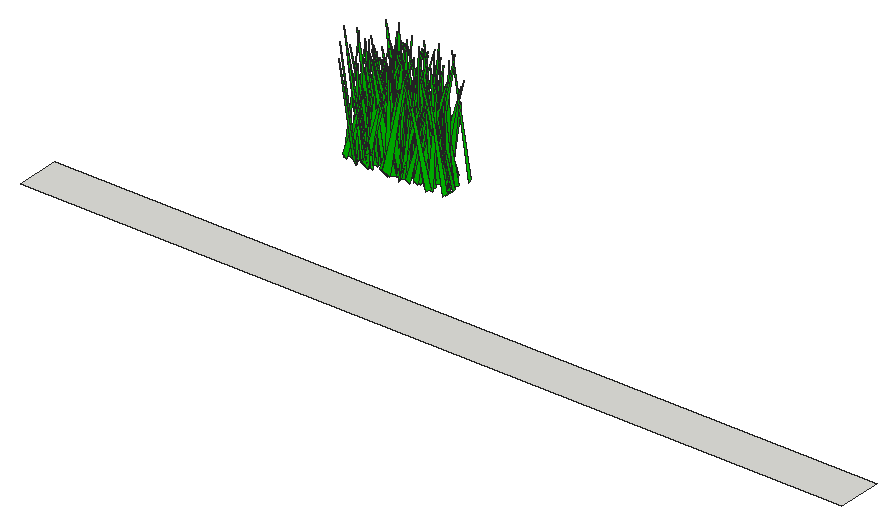
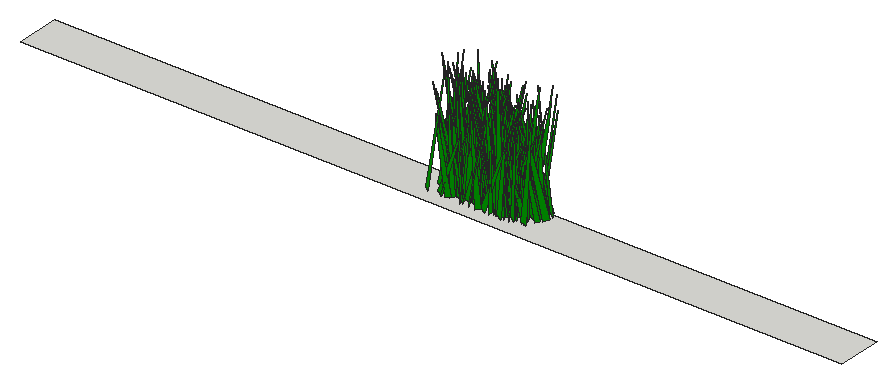
# SketchUp Ruby script. Lengths in inches.
U = 1.inch
M = Sketchup.active_model
def pt(a) = Geom::Point3d.new(a.map { |v| v * U })
def face(e, loops, mat)
  f = e.add_face(loops[0].map { |a| pt(a) })
  loops[1..].each { |l| e.add_face(l.map { |a| pt(a) }).erase! }
  f.material = f.back_material = mat if mat
  f
end
# faces: each face lists its corners as indices into pts; further lists are holes
def faces(e, pts, list, mat = nil) = list.each { |f| face(e, (f[0].is_a?(Array) ? f : [f]).map { |l| l.map { |i| pts[i] } }, mat) }
# xy, xz, yz: faces in a plane at the given z, y or x. An outline is a flat list of corners, or four numbers for a rectangle; further outlines are holes
def ring(l) = l.size == 4 ? [[l[0], l[1]], [l[2], l[1]], [l[2], l[3]], [l[0], l[3]]] : l.each_slice(2).to_a
def flat(e, list, mat, &to3) = list.each { |f| face(e, (f[0].is_a?(Array) ? f : [f]).map { |l| ring(l).map { |u, v| to3.(u, v) } }, mat) }
def xy(e, z, list, mat = nil) = flat(e, list, mat) { |x, y| [x, y, z] }
def xz(e, y, list, mat = nil) = flat(e, list, mat) { |x, z| [x, y, z] }
def yz(e, x, list, mat = nil) = flat(e, list, mat) { |y, z| [x, y, z] }
def lines(e, pts, list) = list.each { |a, b| e.add_line(pt(pts[a]), pt(pts[b])) }
# prism: a flat outline (further loops are holes) pulled along v
def prism(e, loops, v, mat = nil)
  f = face(e, loops, mat); d = Geom::Vector3d.new(v.map { |x| x * U })
  f.pushpull(f.normal.samedirection?(d) ? d.length : -d.length)
end
def box(e, o, s, mat = nil) = prism(e, [[o, [o[0] + s[0], o[1], o[2]], [o[0] + s[0], o[1] + s[1], o[2]], [o[0], o[1] + s[1], o[2]]]], [0, 0, s[2]], mat)
def at(x, y, z, deg = 0) = Geom::Transformation.translation(pt([x, y, z])) * Geom::Transformation.rotation(ORIGIN, Z_AXIS, deg.degrees)
def axes(o, x, y, z) = Geom::Transformation.new([*x, 0, *y, 0, *z, 0, *pt(o).to_a, 1])
def part(name) = M.definitions.add(name)
# library, detail: a bought-in or finely detailed component or shape, given as its bounding box
def library(name, o, s) = part(name).tap { |d| box(d.entities, o, s) }
def detail(e, o, s) = box(e.add_group.entities, o, s)
def put(e, d, t, mat = nil) = e.add_instance(d, t).tap { |i| i.material = mat if mat }
def group(e, t, mat = nil) = e.add_group.tap { |g| g.transformation = t; g.material = mat if mat }.entities
root = M.entities
M.materials.add("[Color G06]").color = [0, 204, 0]
c1 = part("fur_instance\#9")
p = [[0.8125,0,1.79],[0.67,-0.02,1.48],[0,-0.11,0],[0,0.11,0]]
faces(c1.entities,p,[[0,1,2,3]])
xy(root,-6,[[0,2.125,121.48,8.54]])
put(root,c1,axes([37.9,20.02,4.28],[3.47157,-0.40469,2.82087],[-2.71349,-0.54955,-1.5974],[-2.14984,0.04013,6.57137]),"[Color G06]")
put(root,c1,axes([36.61,16.41,4.28],[5.3753,0.40513,1.33326],[2.6238,-0.74616,2.41617],[-1.53363,0.14338,8.80669]),"[Color G06]")
put(root,c1,axes([38.46,16.13,4.28],[-5.34603,-0.33105,0.96487],[-2.04621,0.71785,2.96871],[1.36603,-0.22032,8.22297]),"[Color G06]")
put(root,c1,axes([38.41,15.91,4.28],[-4.47863,-0.33847,0.47927],[-2.21714,0.60022,2.41435],[1.03862,-0.17823,7.22054]),"[Color G06]")
put(root,c1,axes([36.875,16.71,4.28],[2.72341,-0.07354,0.24648],[-0.46764,-0.36835,-1.08371],[-0.29438,-0.09522,4.00182]),"[Color G06]")
put(root,c1,axes([39.02,16.71,4.28],[-5.99343,0.00503,1.97221],[0.37096,0.82741,2.27576],[1.26688,-0.21848,8.66388]),"[Color G06]")
put(root,c1,axes([39.23,16.65,4.28],[1.57209,0.66026,3.05765],[4.59503,-0.31476,2.53052],[-2.34314,-0.17427,7.01397]),"[Color G06]")
put(root,c1,axes([37.36,17.24,4.28],[-1.95487,-0.62971,0.15551],[-4.29388,0.26397,2.21887],[1.40215,-0.06957,7.01177]),"[Color G06]")
put(root,c1,axes([36.71,17.56,4.28],[3.09184,0.18506,0.79522],[1.42073,-0.41751,-1.17771],[-0.16067,-0.13068,4.88882]),"[Color G06]")
put(root,c1,axes([36.69,16.27,4.28],[1.20073,0.42806,0.95635],[2.99606,-0.12842,-1.79969],[0.92537,-0.13966,4.58593]),"[Color G06]")
put(root,c1,axes([36.82,18.85,4.28],[0.9216,-0.47973,0.36918],[-3.30858,-0.11288,1.59852],[0.97464,0.07042,5.07737]),"[Color G06]")
put(root,c1,axes([38.26,19.15,4.28],[-2.20159,0.26204,0.34237],[1.66664,0.29153,-1.69253],[0.89785,0.1014,3.98126]),"[Color G06]")
put(root,c1,axes([37.28,16.53,4.28],[1.57039,-0.41551,1.11701],[-3.05096,-0.19725,1.15225],[0.35942,0.14109,4.90046]),"[Color G06]")
put(root,c1,axes([38.1,19.6,4.28],[1.84083,0.34898,0.07112],[2.41519,-0.2498,1.1692],[-0.65754,0.05947,4.49365]),"[Color G06]")
put(root,c1,axes([39.87,17.3,4.28],[-4.77005,0.24701,1.28332],[1.92796,0.64961,1.6439],[0.39758,-0.18651,7.42509]),"[Color G06]")
put(root,c1,axes([36.17,17.9375,4.28],[1.95013,-0.68167,0.55856],[-4.65744,-0.24007,2.66678],[1.5312,0.13796,7.40016]),"[Color G06]")
put(root,c1,axes([37.83,16.66,4.28],[4.02135,0.43561,1.35126],[3.01311,-0.57451,1.24567],[-1.22366,0.01692,7.50797]),"[Color G06]")
put(root,c1,axes([38.66,18.71,4.28],[2.46337,-0.65775,1.1822],[-4.57502,-0.36023,-1.72948],[-1.39439,0.01991,7.76295]),"[Color G06]")
put(root,c1,axes([37.02,17.84,4.28],[1.06994,-0.42591,0.47783],[-2.8174,-0.11735,2.07629],[1.22202,0.10236,4.36859]),"[Color G06]")
put(root,c1,axes([38.58,18.8,4.28],[4.83292,0.01981,3.5778],[0.91968,-0.7089,-2.32403],[-2.21471,-0.25114,6.84236]),"[Color G06]")
put(root,c1,axes([38.28,18.14,4.28],[3.16808,-0.30182,0.2175],[-1.87489,-0.39902,-2.60553],[-1.09119,-0.19067,5.10835]),"[Color G06]")
put(root,c1,axes([39.37,17,4.28],[-2.99921,-0.13256,0.2159],[-0.79345,0.37846,2.07318],[0.54316,-0.17912,4.22063]),"[Color G06]")
put(root,c1,axes([38.45,19.2,4.28],[-2.28366,0.25573,0.50237],[1.34667,0.2775,-2.55289],[1.28944,0.16309,3.55591]),"[Color G06]")
put(root,c1,axes([40.27,17.23,4.28],[-2.436,-0.68615,3.33008],[-5.38871,0.28525,-2.05343],[-0.37171,0.36132,7.94493]),"[Color G06]")
put(root,c1,axes([41.15,19.15,4.28],[-2.91514,-0.46739,0.51783],[-3.17393,0.3594,-2.64669],[-1.13173,0.19598,6.08874]),"[Color G06]")
put(root,c1,axes([39.55,20.05,4.28],[3.03515,0.37899,1.79669],[2.38162,-0.45351,2.00239],[-1.7776,0.0395,5.75051]),"[Color G06]")
put(root,c1,axes([37.66,19.83,4.28],[1.90811,-0.33101,0.57774],[-2.2249,-0.21682,2.14381],[0.91331,0.16338,4.01546]),"[Color G06]")
put(root,c1,axes([40.06,18.02,4.28],[0.92103,0.36703,1.61141],[2.57058,-0.17506,1.29835],[-1.2175,-0.09195,3.9603]),"[Color G06]")
put(root,c1,axes([38.1875,17.9,4.28],[1.30742,-0.3652,0.60763],[-2.55676,-0.15715,1.43856],[0.69795,0.10843,4.13156]),"[Color G06]")
put(root,c1,axes([40.63,16.73,4.28],[0.77732,0.51302,3.25734],[3.89469,-0.21246,1.7678],[-1.76527,-0.24285,5.3346]),"[Color G06]")
put(root,c1,axes([38.67,17.08,4.28],[3.32335,0.01282,1.22974],[0.40887,-0.43813,-1.94364],[-0.71991,-0.18966,4.57297]),"[Color G06]")
put(root,c1,axes([39.51,19.86,4.28],[2.7249,0.37399,0.82328],[2.36466,-0.37609,2.14307],[-1.38016,0.09403,5.29721]),"[Color G06]")
put(root,c1,axes([40.13,19.0625,4.28],[1.69041,0.66589,0.23381],[4.5076,-0.22994,2.43201],[-1.58412,0.05628,7.16976]),"[Color G06]")
put(root,c1,axes([39.3,17.14,4.28],[1.8635,-0.28338,0.02215],[-1.94834,-0.24992,-1.15234],[-0.57789,-0.0712,3.95651]),"[Color G06]")
put(root,c1,axes([37.42,17.87,4.28],[5.61312,-0.09811,0.53465],[-0.76809,-0.76144,1.96194],[-0.18168,0.18803,8.22408]),"[Color G06]")
put(root,c1,axes([37.83,19.9,4.28],[2.15712,-0.48657,0.05081],[-3.35989,-0.28811,1.6855],[0.94209,0.08657,5.89488]),"[Color G06]")
put(root,c1,axes([40.9,17,4.28],[0.01484,0.62308,0.37127],[4.27676,-0.01217,1.96518],[-1.31769,-0.0325,6.38248]),"[Color G06]")
put(root,c1,axes([39.39,19.71,4.28],[2.78221,0.45022,0.453],[3.15302,-0.38859,1.10803],[-0.75788,0.03613,6.27277]),"[Color G06]")
put(root,c1,axes([41.39,17.46,4.28],[-2.30428,0.59124,0.03106],[4.18614,0.31671,1.16245],[-0.67359,-0.0543,7.11798]),"[Color G06]")
put(root,c1,axes([40.78,19.72,4.28],[0.17621,-0.46232,0.7413],[-3.19427,-0.04417,-1.46832],[-1.01708,0.05862,4.73986]),"[Color G06]")
put(root,c1,axes([39.56,20.57,4.28],[3.23098,0.03977,1.39197],[0.4922,-0.45493,-1.05907],[-0.84051,-0.11355,4.73061]),"[Color G06]")
put(root,c1,axes([40.38,20.42,4.28],[-4.109,-0.25493,1.46449],[-1.28515,0.5509,2.96169],[1.62809,-0.20853,6.03392]),"[Color G06]")
put(root,c1,axes([41.3125,17.96,4.28],[-1.79413,-0.37217,0.82138],[-2.70437,0.23194,-1.12229],[-0.3341,0.12111,4.67356]),"[Color G06]")
put(root,c1,axes([40.97,15.92,4.28],[-3.25958,0.1412,0.88958],[0.85784,0.45342,-1.24648],[0.80234,0.08886,4.94671]),"[Color G06]")
put(root,c1,axes([38.86,19.08,4.28],[5.4935,-0.05604,1.30425],[-0.56977,-0.75877,1.61586],[-0.77354,0.16094,8.07224]),"[Color G06]")
put(root,c1,axes([38.04,16.74,4.28],[4.01598,-0.35896,0.20669],[-2.44461,-0.51896,2.56565],[0.81813,0.21133,6.6517]),"[Color G06]")
put(root,c1,axes([40.79,18.12,4.28],[1.14185,-0.43327,0.18231],[-2.96496,-0.15717,-1.42682],[-0.93697,-0.03066,4.73722]),"[Color G06]")
put(root,c1,axes([42.55,19.83,4.28],[-2.61322,0.43396,0.9154],[2.93762,0.28943,2.97089],[-1.19593,-0.23731,5.29728]),"[Color G06]")
put(root,c1,axes([40.98,20.67,4.28],[-5.07749,0.20615,3.40636],[2.13672,0.71909,2.11516],[1.67766,-0.29193,7.61553]),"[Color G06]")
put(root,c1,axes([39.05,18.68,4.28],[2.60853,-0.30912,0.97826],[-2.22361,-0.29805,2.42559],[0.63084,0.22761,4.50473]),"[Color G06]")
put(root,c1,axes([40.03,19.88,4.28],[-0.88113,0.73929,2.82344],[5.50689,0.1683,-1.22356],[1.16214,-0.23699,7.93868]),"[Color G06]")
put(root,c1,axes([40.32,19.27,4.28],[5.24783,0.16053,2.27414],[0.66127,-0.73549,2.55543],[-1.78976,0.19895,7.61229]),"[Color G06]")
put(root,c1,axes([40.29,16.29,4.28],[-1.46176,0.70455,0.83502],[4.91638,0.21655,-1.76494],[1.29207,-0.02691,7.66036]),"[Color G06]")
put(root,c1,axes([42.14,16.95,4.28],[-2.29832,0.49842,1.35675],[3.66913,0.29408,1.4735],[-0.37039,-0.1796,6.17784]),"[Color G06]")
put(root,c1,axes([40.77,16.88,4.28],[-1.34688,-0.47136,0.37153],[-3.30429,0.19091,1.06667],[0.75478,-0.00535,5.33271]),"[Color G06]")
put(root,c1,axes([40.93,19.24,4.28],[2.39903,0.4259,0.68473],[2.92901,-0.33941,1.3284],[-0.97931,0.02818,5.65051]),"[Color G06]")
put(root,c1,axes([39.1875,19,4.28],[4.33206,0.52704,0.98439],[3.83529,-0.59146,-1.32475],[0.09616,-0.1534,8.48964]),"[Color G06]")
put(root,c1,axes([40.98,19.04,4.28],[-2.03549,0.63209,0.25757],[4.38551,0.28095,-1.78624],[1.15945,0.04703,7.20845]),"[Color G06]")
put(root,c1,axes([40.875,17.68,4.28],[3.09695,0.16286,1.11518],[0.96393,-0.43613,1.3373],[-0.99582,0.08433,4.76264]),"[Color G06]")
put(root,c1,axes([41,20.5,4.28],[-1.8805,-0.8159,1.88088],[-5.85758,0.28865,1.30182],[1.22764,0.12745,9.09264]),"[Color G06]")
put(root,c1,axes([40.03,15.99,4.28],[0.89705,-0.54544,0.81967],[-3.80481,-0.09828,1.78834],[1.0601,0.10879,5.72493]),"[Color G06]")
put(root,c1,axes([42.34,18.75,4.28],[-3.97404,0.10676,1.49318],[1.04291,0.53761,1.78475],[0.70468,-0.1936,5.7794]),"[Color G06]")
put(root,c1,axes([39.95,15.94,4.28],[0.37594,-0.45159,2.36028],[-3.31276,0.04374,2.14],[1.41677,0.2221,4.37754]),"[Color G06]")
put(root,c1,axes([41.29,17.07,4.28],[-1.34818,0.33315,0.10678],[2.28213,0.18282,-1.16105],[0.71046,0.04493,3.93215]),"[Color G06]")
put(root,c1,axes([41.64,18.4,4.28],[-3.24505,0.30939,3.63929],[3.03712,0.46558,1.50235],[1.27588,-0.32138,5.67989]),"[Color G06]")
put(root,c1,axes([38.54,17.39,4.28],[2.26184,-0.80096,0.72185],[-5.30689,-0.26112,3.86036],[2.24991,0.18929,8.3798]),"[Color G06]")
put(root,c1,axes([43.04,19.35,4.28],[-3.87817,0.66668,1.77878],[4.92534,0.52988,1.17285],[0.12292,-0.19805,9.12571]),"[Color G06]")
put(root,c1,axes([43.22,17.3,4.28],[-2.48583,0.47756,0.74619],[3.40039,0.32105,1.70001],[-0.64443,-0.14809,6.09197]),"[Color G06]")
put(root,c1,axes([43.45,18.9,4.28],[-3.03107,0.57663,1.47437],[4.21376,0.38514,2.0469],[-0.56284,-0.22189,7.38433]),"[Color G06]")
put(root,c1,axes([40.54,20.15,4.28],[-0.16569,-0.67927,0.67506],[-4.69176,0.03992,2.04153],[1.38576,0.05392,6.99271]),"[Color G06]")
put(root,c1,axes([43.53,20.47,4.28],[-2.26695,0.4404,0.49521],[3.02675,0.28248,2.09162],[-0.96078,-0.14923,5.42081]),"[Color G06]")
put(root,c1,axes([43.64,16.79,4.28],[-6.0251,-0.10159,1.28],[-0.92291,0.81868,-2.23967],[0.64224,0.2234,8.78969]),"[Color G06]")
put(root,c1,axes([41.65,19.39,4.28],[4.52778,-0.00816,2.8291],[-0.4034,-0.67251,1.21946],[-1.85036,0.12666,6.65689]),"[Color G06]")
put(root,c1,axes([44.22,17.91,4.28],[-5.06046,0.2296,0.55738],[1.65502,0.64223,3.17323],[-0.33335,-0.29698,7.29309]),"[Color G06]")
put(root,c1,axes([39.7,18.25,4.28],[3.54743,-0.62754,2.24139],[-4.66804,-0.41542,3.14228],[0.8431,0.34039,7.96711]),"[Color G06]")
put(root,c1,axes([42.01,17.27,4.28],[-2.01232,-0.33381,0.42476],[-2.24635,0.27839,1.36062],[0.87469,-0.053,4.4715]),"[Color G06]")
put(root,c1,axes([43.92,15.98,4.28],[-1.41782,0.76513,0.18827],[5.29749,0.18604,2.26136],[-1.43492,-0.06919,8.16253]),"[Color G06]")
put(root,c1,axes([42.4,17.5625,4.28],[-3.54438,0.03855,2.05396],[-0.38921,0.47351,-2.52124],[1.34669,0.23832,4.67717]),"[Color G06]")
put(root,c1,axes([41.88,19.04,4.28],[-3.24261,0.74246,0.53827],[4.91756,0.43854,-3.31536],[2.0728,0.12108,8.70748]),"[Color G06]")
put(root,c1,axes([42.26,20.67,4.28],[-3.02277,-0.30402,1.64311],[-1.88164,0.44552,1.73704],[1.55603,-0.05184,5.29246]),"[Color G06]")
put(root,c1,axes([42.31,19.19,4.28],[2.6441,0.32077,0.92856],[2.15184,-0.37704,1.27494],[-1.02327,0.03599,5.08046]),"[Color G06]")
put(root,c1,axes([44.85,18.77,4.28],[-4.61999,-0.20153,0.10743],[-1.35404,0.59028,-2.86944],[-0.51028,0.25829,6.64151]),"[Color G06]")
put(root,c1,axes([44.47,16.875,4.28],[-4.02108,-0.56871,1.03129],[-4.12362,0.54064,-1.6662],[-0.32442,0.17714,8.39621]),"[Color G06]")
put(root,c1,axes([42.2,19.99,4.28],[3.7176,0.69653,0.00145],[4.84541,-0.50292,2.25944],[-1.2133,0.12576,9.02767]),"[Color G06]")
put(root,c1,axes([41.13,18.48,4.28],[4.23005,-0.0028,0.25051],[-0.05377,-0.57795,1.28674],[-0.16001,0.12026,6.18986]),"[Color G06]")
put(root,c1,axes([42.24,19.625,4.28],[3.41911,-0.16408,1.25206],[-1.01031,-0.4862,-1.15657],[-1.03228,-0.06761,5.27904]),"[Color G06]")
put(root,c1,axes([43.1,18.3,4.28],[-2.27319,0.52855,0.1698],[3.70692,0.31362,-1.29214],[0.79899,0.0487,6.47802]),"[Color G06]")
put(root,c1,axes([45.3,16.38,4.28],[-2.15665,-0.72692,2.03688],[-5.12725,0.21394,-3.35565],[-1.65641,0.28423,7.73506]),"[Color G06]")
put(root,c1,axes([41.27,19.46,4.28],[3.0794,0.44815,0.29743],[3.17147,-0.4155,-1.42896],[0.55656,-0.1119,6.49701]),"[Color G06]")
put(root,c1,axes([45.1,18.32,4.28],[-4.97733,0.16058,0.36025],[1.17635,0.6819,1.38728],[0.02146,-0.13369,7.50842]),"[Color G06]")
put(root,c1,axes([42.27,20.07,4.28],[4.07211,0.16064,0.99922],[0.96312,-0.56227,1.61655],[-0.92004,0.1224,6.11484]),"[Color G06]")
put(root,c1,axes([43.63,19.33,4.28],[1.32383,-0.54452,1.68483],[-3.90365,-0.21638,-1.18183],[-1.13159,0.10941,6.04802]),"[Color G06]")
put(root,c1,axes([44.32,19.12,4.28],[0.42983,-0.57936,2.2609],[-4.19174,-0.12083,-1.77681],[-1.40692,0.183,5.98449]),"[Color G06]")
put(root,c1,axes([41.6,19.9375,4.28],[3.90604,-0.42439,0.62813],[-3.07041,-0.53588,1.05735],[0.10826,0.11375,7.32481]),"[Color G06]")
put(root,c1,axes([43.01,17.38,4.28],[5.17048,-0.00353,3.15679],[0.60247,-0.74398,-2.29981],[-2.02458,-0.23041,7.3776]),"[Color G06]")
put(root,c1,axes([43.14,16.2,4.28],[2.64687,-0.61369,1.05599],[-4.34877,-0.38069,-1.06597],[-0.97758,0.03187,7.60113]),"[Color G06]")
put(root,c1,axes([43.48,18.27,4.28],[4.44366,-0.60121,0.48089],[-3.74938,-0.56792,-4.17236],[-2.15272,-0.25188,8.25962]),"[Color G06]")
put(root,c1,axes([42.27,19.95,4.28],[3.38657,0.22648,0.63089],[1.67699,-0.46164,-1.07044],[-0.06196,-0.11561,5.51047]),"[Color G06]")
put(root,c1,axes([42.71,16.05,4.28],[1.36146,0.52195,1.16092],[3.79982,-0.17218,-1.06133],[0.41866,-0.13465,5.85748]),"[Color G06]")
put(root,c1,axes([43.69,17.62,4.28],[4.94173,-0.22195,4.25139],[-2.35354,-0.74137,1.66469],[-2.25516,0.28735,7.57876]),"[Color G06]")
put(root,c1,axes([42.01,19.8,4.28],[5.36927,0.04607,0.69987],[0.10303,-0.68284,3.39765],[-0.56374,0.31397,7.28674]),"[Color G06]")
put(root,c1,axes([44.1875,16.59,4.28],[-4.04709,-0.34153,3.08183],[-2.92871,0.58216,-1.17973],[1.29356,0.24951,6.97097]),"[Color G06]")
put(root,c1,axes([46.66,19.31,4.28],[-3.24904,-0.73428,0.39636],[-4.9902,0.41425,-3.21497],[-1.70177,0.18716,8.67069]),"[Color G06]")
put(root,c1,axes([42.57,17.14,4.28],[-0.27933,-0.82853,2.61803],[-6.00069,0.09687,2.09164],[1.53725,0.22759,8.64046]),"[Color G06]")
put(root,c1,axes([42.0625,19.91,4.28],[5.34742,-0.17193,1.50877],[-1.54727,-0.6781,3.37281],[-0.38113,0.34062,7.47621]),"[Color G06]")
put(root,c1,axes([43.9375,19.25,4.28],[3.41881,-0.5942,0.58715],[-3.978,-0.46715,-2.56819],[-1.57711,-0.10978,7.75063]),"[Color G06]")
put(root,c1,axes([42.42,19.71,4.28],[4.59203,0.09908,0.27075],[0.66364,-0.6297,1.33029],[-0.31192,0.11896,6.8162]),"[Color G06]")
put(root,c1,axes([44.84,16.47,4.28],[-5.33125,-0.17683,2.051],[-1.08906,0.7642,1.2452],[1.51827,-0.07275,8.09503]),"[Color G06]")
put(root,c1,axes([45.37,20.75,4.28],[-5.10601,-0.09108,1.31939],[-0.45333,0.70807,1.69605],[1.0002,-0.14402,7.50421]),"[Color G06]")
put(root,c1,axes([46.35,19.87,4.28],[-4.94522,0.33322,0.58279],[2.42115,0.67968,1.24894],[-0.01748,-0.12857,8.11308]),"[Color G06]")
put(root,c1,axes([42.49,16.09,4.28],[-0.77698,0.63143,3.11383],[4.35047,0.22942,-2.91929],[2.43274,-0.20859,6.21509]),"[Color G06]")
put(root,c1,axes([43,15.97,4.28],[1.73406,0.66096,1.84019],[4.83908,-0.20329,-1.79818],[0.75221,-0.21592,7.32584]),"[Color G06]")
put(root,c1,axes([43.27,18.64,4.28],[-0.22271,0.80024,1.56894],[5.63797,0.06717,-2.14818],[1.49945,-0.13372,8.31025]),"[Color G06]")
put(root,c1,axes([44.59,19.45,4.28],[3.58768,-0.01203,2.73155],[-0.69378,-0.52802,1.7683],[-1.69304,0.19088,5.06373]),"[Color G06]")
put(root,c1,axes([42.96,19.5,4.28],[4.56969,-0.41445,1.953],[-3.23629,-0.60664,2.12621],[-0.25984,0.26692,7.8649]),"[Color G06]")
put(root,c1,axes([43.625,17.98,4.28],[4.12255,-0.10445,0.93885],[-0.60627,-0.57099,-1.3509],[-0.76689,-0.11011,6.11489]),"[Color G06]")
put(root,c1,axes([44.32,16.61,4.28],[3.64534,-0.34719,0.85169],[-2.18828,-0.49595,-2.30304],[-1.31728,-0.13691,6.18274]),"[Color G06]")
put(root,c1,axes([44.4,17.09,4.28],[-3.32519,0.6309,2.44718],[4.47653,0.5074,-1.43979],[1.76388,-0.09838,8.26735]),"[Color G06]")
put(root,c1,axes([43.17,18.5625,4.28],[5.04705,-0.3478,2.19253],[-2.83519,-0.67661,2.24882],[-0.57844,0.28172,8.10792]),"[Color G06]")
put(root,c1,axes([45.52,18.38,4.28],[-5.12642,-0.39395,0.02862],[-2.44156,0.62055,4.35669],[1.4215,-0.35489,7.58625]),"[Color G06]")
put(root,c1,axes([42.24,19.79,4.28],[5.94338,0.19193,0.22752],[1.3825,-0.81702,-1.49558],[0.07954,-0.14071,8.99442]),"[Color G06]")
put(root,c1,axes([42.86,18.49,4.28],[3.41535,-0.52846,0.93964],[-3.80291,-0.44852,1.89873],[0.54323,0.18257,7.38457]),"[Color G06]")
put(root,c1,axes([45.42,17.24,4.28],[0.85938,0.68296,2.37864],[5.02864,-0.1598,1.21254],[-1.11039,-0.19513,7.33219]),"[Color G06]")
put(root,c1,axes([45.43,17.12,4.28],[-2.90777,0.16196,0.31626],[1.0244,0.38512,-1.61804],[0.5869,0.13024,4.39113]),"[Color G06]")
put(root,c1,axes([44.44,17.34,4.28],[-3.41484,-0.2633,1.71396],[-0.97239,0.4435,3.49891],[1.98363,-0.23586,4.66577]),"[Color G06]")
put(root,c1,axes([43.51,18.9,4.28],[5.49781,0.02598,1.73774],[0.60057,-0.72776,-2.99441],[-1.01287,-0.2905,7.6569]),"[Color G06]")
put(root,c1,axes([44.93,20.1,4.28],[2.113,0.48748,0.94715],[3.41127,-0.3071,1.15791],[-0.99283,-0.0177,5.99423]),"[Color G06]")
put(root,c1,axes([44.07,20.71,4.28],[-0.76323,-0.67811,0.15171],[-4.69089,0.10641,1.92206],[1.28594,-0.01431,7.10142]),"[Color G06]")
put(root,c1,axes([45.12,18.37,4.28],[-2.08718,-0.25782,0.7248],[-1.67961,0.29518,1.25746],[0.91235,-0.04639,3.97308]),"[Color G06]")
put(root,c1,axes([47.49,19.63,4.28],[-1.6465,0.74365,2.04473],[5.23821,0.15029,3.14301],[-1.695,-0.25792,7.72691]),"[Color G06]")
put(root,c1,axes([48.5,17.78,4.28],[-4.20763,-0.62681,0.93692],[-4.2515,0.50264,-4.01981],[-1.58836,0.31504,8.27774]),"[Color G06]")
put(root,c1,axes([45.49,19.67,4.28],[-2.81552,-0.34408,1.48173],[-2.23762,0.41534,1.58189],[1.43683,-0.02742,5.36705]),"[Color G06]")
put(root,c1,axes([46.15,18.44,4.28],[1.4045,-0.70283,1.71877],[-5.05626,-0.22138,-1.16962],[-1.07708,0.12275,7.73196]),"[Color G06]")
put(root,c1,axes([45.09,15.89,4.28],[5.14713,-0.0828,1.98545],[-0.18775,-0.71305,-2.32866],[-1.44293,-0.20257,7.38536]),"[Color G06]")
put(root,c1,axes([45.96,18.48,4.28],[-2.97762,0.03491,1.91639],[-0.18613,0.42914,-1.54406],[1.29312,0.14216,4.19057]),"[Color G06]")
put(root,c1,axes([45.57,17.1,4.28],[-3.66502,-0.38632,2.08101],[-2.33543,0.54169,2.36405],[2.0395,-0.07394,6.4467]),"[Color G06]")
put(root,c1,axes([46.52,16.86,4.28],[-4.1945,0.16176,1.34899],[0.70533,0.55544,-2.75214],[1.2895,0.22236,5.89337]),"[Color G06]")
put(root,c1,axes([46.7,18.5625,4.28],[1.33707,-0.5079,2.52741],[-3.76075,-0.24552,-1.22382],[-1.40815,0.17346,5.6683]),"[Color G06]")
put(root,c1,axes([44.42,17.64,4.28],[2.1682,-0.53321,1.44056],[-3.85436,-0.25415,2.15224],[0.83324,0.21187,6.20721]),"[Color G06]")
put(root,c1,axes([46.73,20.61,4.28],[-5.66782,-0.30329,1.8466],[-1.67646,0.77726,3.17113],[1.85653,-0.22406,8.50109]),"[Color G06]")
put(root,c1,axes([45.47,16.52,4.28],[3.39374,0.56615,0.5916],[3.99688,-0.47585,1.09615],[-0.8157,0.02383,7.83239]),"[Color G06]")
put(root,c1,axes([45.3,16.22,4.28],[3.65521,-0.34135,0.34816],[-2.36381,-0.5038,-1.3086],[-0.67758,-0.08387,6.44339]),"[Color G06]")
put(root,c1,axes([44.76,16.125,4.28],[2.51275,0.43557,0.30796],[3.07628,-0.33677,-1.35093],[0.57939,-0.10092,5.83719]),"[Color G06]")
put(root,c1,axes([46.76,19.47,4.28],[-3.23734,-0.5208,0.50352],[-3.59293,0.44855,1.69488],[1.07368,-0.06927,7.18994]),"[Color G06]")
put(root,c1,axes([46.64,17.29,4.28],[3.4647,-0.29796,1.96319],[-1.74504,-0.51072,-2.02511],[-1.80164,-0.07832,5.73688]),"[Color G06]")
put(root,c1,axes([47.125,19.9,4.28],[0.51912,0.52243,1.13229],[3.69079,-0.09624,1.32116],[-0.9941,-0.08449,5.49635]),"[Color G06]")
put(root,c1,axes([43.59,17.8,4.28],[4.23344,-0.38895,0.42198],[-2.50339,-0.49235,3.96791],[1.26208,0.32807,6.45505]),"[Color G06]")
put(root,c1,axes([43.875,18.43,4.28],[2.45557,-0.55246,1.18464],[-3.59291,-0.23942,3.80975],[1.84815,0.2686,5.83238]),"[Color G06]")
put(root,c1,axes([46.74,19.03,4.28],[2.36437,-0.76398,0.80235],[-5.3893,-0.33785,-1.47945],[-1.1223,0.01287,8.79468]),"[Color G06]")
put(root,c1,axes([46.07,16.875,4.28],[3.20891,-0.15609,0.29711],[-0.91819,-0.40478,-2.27658],[-0.67034,-0.19274,4.54059]),"[Color G06]")
put(root,c1,axes([45.55,17.35,4.28],[4.24225,-0.03672,0.7265],[-0.16256,-0.5842,-1.27178],[-0.5284,-0.11509,6.22395]),"[Color G06]")
put(root,c1,axes([45.03,19.41,4.28],[5.83473,-0.02957,0.87155],[-0.0918,-0.80163,-1.75112],[-0.61366,-0.16119,8.54868]),"[Color G06]")
put(root,c1,axes([48.35,16.71,4.28],[-1.55112,0.42318,0.19544],[2.95705,0.20569,1.26191],[-0.69471,-0.06935,4.93498]),"[Color G06]")
put(root,c1,axes([44.77,19.44,4.28],[2.1042,0.5545,1.27576],[3.71501,-0.20751,-3.3261],[1.65515,-0.23917,5.84362]),"[Color G06]")
put(root,c1,axes([46.66,19.37,4.28],[3.9883,0.65286,1.15485],[4.58082,-0.56644,1.44786],[-1.23806,0.00729,9.07733]),"[Color G06]")
put(root,c1,axes([47.04,16.75,4.28],[5.52937,0.16592,3.87833],[1.65625,-0.82891,-1.20088],[-2.32516,-0.19587,8.3675]),"[Color G06]")
put(root,c1,axes([49.32,15.93,4.28],[-5.46441,0.3752,1.3203],[2.82597,0.73988,1.97229],[0.18465,-0.21994,8.88714]),"[Color G06]")
put(root,c1,axes([46.57,20.49,4.28],[4.06915,-0.17524,0.98238],[-0.97623,-0.54812,-2.19958],[-1.02876,-0.17303,5.97295]),"[Color G06]")
put(root,c1,axes([46.83,16.61,4.28],[2.58144,-0.31745,0.13352],[-2.18714,-0.35058,-1.29433],[-0.63784,-0.08263,4.97859]),"[Color G06]")
put(root,c1,axes([48.66,18.83,4.28],[-1.0319,-0.48317,0.79733],[-3.41186,0.12058,-1.46967],[-0.80611,0.10817,5.19971]),"[Color G06]")
put(root,c1,axes([46.14,16.05,4.28],[2.75053,0.40097,0.4747],[2.87533,-0.37217,-1.1021],[0.31882,-0.10275,5.84413]),"[Color G06]")
put(root,c1,axes([49.22,17.98,4.28],[0.94702,0.69698,3.07944],[4.95797,-0.22827,2.52911],[-2.15553,-0.21882,7.17019]),"[Color G06]")
put(root,c1,axes([47.45,18.01,4.28],[3.83614,-0.51653,0.55771],[-3.43442,-0.51984,-2.53795],[-1.43689,-0.1365,7.55508]),"[Color G06]")
put(root,c1,axes([46.64,20.31,4.28],[1.41103,0.40657,1.31739],[2.98842,-0.15858,-1.52768],[0.58917,-0.16933,4.59372]),"[Color G06]")
put(root,c1,axes([47.28,20.05,4.28],[3.39695,-0.54627,0.17688],[-3.78716,-0.46314,-1.84614],[-1.00877,-0.10077,7.52643]),"[Color G06]")
put(root,c1,axes([48.31,17.39,4.28],[0.96537,-0.73578,0.41121],[-5.18027,-0.13948,-1.50446],[-1.04012,0.01177,7.87457]),"[Color G06]")
put(root,c1,axes([49.1875,20.35,4.28],[-3.15485,0.14359,0.46031],[1.0646,0.39915,1.99492],[-0.14789,-0.1899,4.5411]),"[Color G06]")
put(root,c1,axes([46.02,17.45,4.28],[4.58826,0.16738,0.82468],[1.32106,-0.58288,-2.82773],[-0.00742,-0.27482,6.49981]),"[Color G06]")
put(root,c1,axes([47.84,19.1,4.28],[-2.97471,-0.74642,0.79778],[-5.17573,0.42032,2.06685],[1.46596,-0.03065,8.91608]),"[Color G06]")
put(root,c1,axes([47.01,16.49,4.28],[0.68131,-0.44533,0.79667],[-3.15325,-0.07402,1.27062],[0.73507,0.09525,4.71219]),"[Color G06]")
put(root,c1,axes([47.9,19.77,4.28],[-2.73194,-0.14559,1.54182],[-0.61455,0.38949,1.79249],[1.33288,-0.11882,3.98665]),"[Color G06]")
put(root,c1,axes([47.65,17.84,4.28],[-1.03933,0.34872,0.86404],[2.39502,0.16304,-1.12364],[0.92304,-0.03038,3.88844]),"[Color G06]")
put(root,c1,axes([46.83,18.15,4.28],[1.92166,-0.52824,0.59965],[-3.76989,-0.25472,1.20964],[0.54682,0.10027,6.23217]),"[Color G06]")
put(root,c1,axes([49.25,18.8,4.28],[-3.46616,0.1729,0.03103],[1.20452,0.47146,-1.22381],[0.29486,0.10656,5.36408]),"[Color G06]")
put(root,c1,axes([46.07,17.54,4.28],[2.24673,0.75348,1.17728],[5.31338,-0.27427,-2.48511],[1.25921,-0.18707,8.38563]),"[Color G06]")
put(root,c1,axes([48.1,20.35,4.28],[-2.76969,0.41906,1.70904],[2.87649,0.41697,-1.33222],[1.43692,-0.02696,5.96108]),"[Color G06]")
put(root,c1,axes([48.17,18.63,4.28],[-2.32838,0.3031,0.85903],[1.89762,0.32681,-1.75724],[1.20575,0.07095,4.4244]),"[Color G06]")
put(root,c1,axes([48.21,18.26,4.28],[4.7113,0.3794,1.21593],[2.00104,-0.59946,4.1678],[-2.01502,0.29177,6.98184]),"[Color G06]")
put(root,c1,axes([48.36,16.89,4.28],[3.65334,-0.15631,3.08205],[-1.63677,-0.55097,1.12377],[-1.68228,0.1966,5.59979]),"[Color G06]")
put(root,c1,axes([49.85,20.54,4.28],[-1.49382,-0.39408,1.00503],[-2.74653,0.15725,-2.03582],[-0.94632,0.1657,4.32208]),"[Color G06]")
put(root,c1,axes([48.18,19.72,4.28],[3.06581,-0.59936,1.13726],[-4.2255,-0.44003,-1.19537],[-1.09464,0.01995,7.79955]),"[Color G06]")
put(root,c1,axes([46.41,17.11,4.28],[4.83812,-0.31236,0.21212],[-2.21647,-0.65749,1.70487],[0.35362,0.15252,7.78382]),"[Color G06]")
put(root,c1,axes([48.72,18.76,4.28],[-1.98959,-0.26355,0.52216],[-1.70031,0.27404,1.41733],[0.8961,-0.06516,3.84867]),"[Color G06]")
put(root,c1,axes([49.09,17.93,4.28],[2.34814,-0.67495,1.36148],[-4.71063,-0.34885,-1.71913],[-1.43804,0.04064,7.85453]),"[Color G06]")
put(root,c1,axes([49.45,20.63,4.28],[-3.07308,-0.31334,0.06881],[-2.13225,0.4099,1.70928],[0.71054,-0.12513,5.42699]),"[Color G06]")
put(root,c1,axes([48.55,19.47,4.28],[-2.92173,0.32031,1.91405],[2.00564,0.44405,-1.69761],[1.70113,0.02661,5.28891]),"[Color G06]")
put(root,c1,axes([48.62,17.375,4.28],[-3.6194,0.46487,1.06389],[2.66846,0.47647,-3.63794],[2.12127,0.19381,6.39163]),"[Color G06]")
put(root,c1,axes([49.48,16.6,4.28],[2.88853,-0.5038,0.38989],[-3.2191,-0.37836,-2.89021],[-1.66079,-0.14285,6.2802]),"[Color G06]")
put(root,c1,axes([47.15,16.75,4.28],[3.37964,0.61927,0.13412],[4.37341,-0.46117,-1.55853],[0.77654,-0.09786,8.19379]),"[Color G06]")
put(root,c1,axes([47.47,18.36,4.28],[6.12856,-0.13103,1.49797],[-1.14765,-0.83949,2.05274],[-0.75523,0.21242,9.0364]),"[Color G06]")
put(root,c1,axes([48.24,19.04,4.28],[0.76418,-0.44354,0.79402],[-3.1219,-0.08267,1.40662],[0.80824,0.10005,4.68245]),"[Color G06]")
put(root,c1,axes([51.67,16.67,4.28],[-4.44391,-0.48132,1.40247],[-3.52762,0.5552,-3.07994],[-0.59196,0.30477,7.82558]),"[Color G06]")
put(root,c1,axes([47.74,18.53,4.28],[3.96033,0.54279,2.05814],[4.12862,-0.51733,-2.07286],[0.05066,-0.27245,8.03635]),"[Color G06]")
put(root,c1,axes([48.59,20.6,4.28],[0.72989,-0.50018,0.83014],[-3.54338,-0.08106,1.34843],[0.78689,0.09893,5.30204]),"[Color G06]")
put(root,c1,axes([50.04,18.16,4.28],[-5.75011,-0.10363,3.1802],[-0.2741,0.83918,2.03427],[2.23715,-0.16354,8.42328]),"[Color G06]")
put(root,c1,axes([49.4,16.15,4.28],[-3.41306,0.36482,2.76963],[2.50699,0.53896,-1.25423],[1.99839,-0.05305,6.30371]),"[Color G06]")
put(root,c1,axes([51.64,17.76,4.28],[-3.95823,-0.23233,0.85458],[-1.75897,0.51087,-2.24425],[-0.09395,0.22368,6.01343]),"[Color G06]")
put(root,c1,axes([48.59,18.75,4.28],[-1.15989,0.71165,0.07231],[4.67314,0.15087,-3.12923],[2.05157,0.05868,7.16874]),"[Color G06]")
put(root,c1,axes([48.375,19.24,4.28],[4.95108,0.19264,0.30879],[1.32115,-0.68027,1.43335],[-0.45346,0.12131,7.5475]),"[Color G06]")
put(root,c1,axes([49.78,18.95,4.28],[-3.27514,-0.62874,2.17653],[-4.41774,0.49445,1.55889],[1.71297,0.07305,8.18182]),"[Color G06]")
put(root,c1,axes([50.89,16.92,4.28],[-3.16697,0.05135,0.64663],[0.23233,0.42884,-1.37043],[0.51847,0.1215,4.56385]),"[Color G06]")
put(root,c1,axes([51.43,16.32,4.28],[-5.10568,0.17085,1.75681],[1.48101,0.70215,1.77027],[0.83032,-0.20185,7.64517]),"[Color G06]")
put(root,c1,axes([51.34,17.18,4.28],[-5.97003,-0.15752,2.05058],[-0.85962,0.84284,1.84739],[1.5555,-0.1388,8.89108]),"[Color G06]")
put(root,c1,axes([51.19,18.89,4.28],[-0.16365,0.3715,0.73519],[2.59254,0.00153,1.20019],[-0.78626,-0.07227,3.80439]),"[Color G06]")
put(root,c1,axes([50.76,18.16,4.28],[1.07421,-0.55498,0.4826],[-3.91523,-0.15555,-1.08213],[-0.784,0.01641,6.0653]),"[Color G06]")
put(root,c1,axes([51.72,20.65,4.28],[-5.68208,0.07309,2.08001],[0.84642,0.78916,1.97929],[1.22277,-0.20662,8.29548]),"[Color G06]")
put(root,c1,axes([49.55,19.29,4.28],[-0.27555,-0.62588,0.35696],[-4.32434,0.04601,1.81172],[1.22572,0.02164,6.47199]),"[Color G06]")
